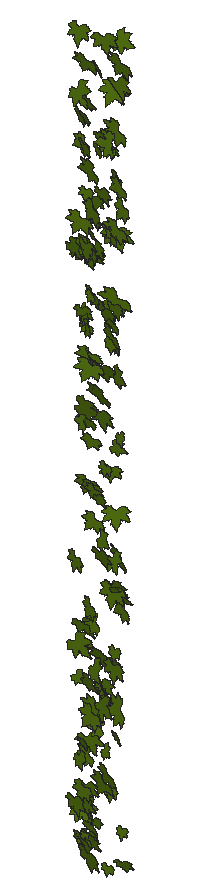
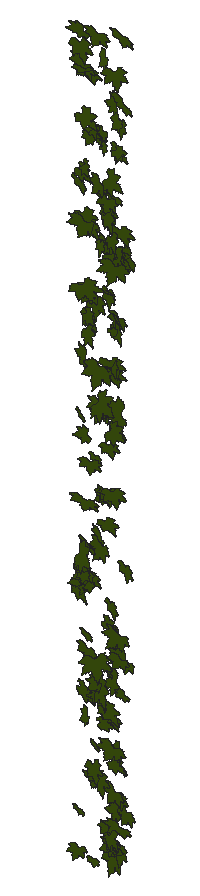
# SketchUp Ruby script. Lengths in inches.
U = 1.inch
M = Sketchup.active_model
def pt(a) = Geom::Point3d.new(a.map { |v| v * U })
def face(e, loops, mat)
  f = e.add_face(loops[0].map { |a| pt(a) })
  loops[1..].each { |l| e.add_face(l.map { |a| pt(a) }).erase! }
  f.material = f.back_material = mat if mat
  f
end
# faces: each face lists its corners as indices into pts; further lists are holes
def faces(e, pts, list, mat = nil) = list.each { |f| face(e, (f[0].is_a?(Array) ? f : [f]).map { |l| l.map { |i| pts[i] } }, mat) }
# xy, xz, yz: faces in a plane at the given z, y or x. An outline is a flat list of corners, or four numbers for a rectangle; further outlines are holes
def ring(l) = l.size == 4 ? [[l[0], l[1]], [l[2], l[1]], [l[2], l[3]], [l[0], l[3]]] : l.each_slice(2).to_a
def flat(e, list, mat, &to3) = list.each { |f| face(e, (f[0].is_a?(Array) ? f : [f]).map { |l| ring(l).map { |u, v| to3.(u, v) } }, mat) }
def xy(e, z, list, mat = nil) = flat(e, list, mat) { |x, y| [x, y, z] }
def xz(e, y, list, mat = nil) = flat(e, list, mat) { |x, z| [x, y, z] }
def yz(e, x, list, mat = nil) = flat(e, list, mat) { |y, z| [x, y, z] }
def lines(e, pts, list) = list.each { |a, b| e.add_line(pt(pts[a]), pt(pts[b])) }
# prism: a flat outline (further loops are holes) pulled along v
def prism(e, loops, v, mat = nil)
  f = face(e, loops, mat); d = Geom::Vector3d.new(v.map { |x| x * U })
  f.pushpull(f.normal.samedirection?(d) ? d.length : -d.length)
end
def box(e, o, s, mat = nil) = prism(e, [[o, [o[0] + s[0], o[1], o[2]], [o[0] + s[0], o[1] + s[1], o[2]], [o[0], o[1] + s[1], o[2]]]], [0, 0, s[2]], mat)
def at(x, y, z, deg = 0) = Geom::Transformation.translation(pt([x, y, z])) * Geom::Transformation.rotation(ORIGIN, Z_AXIS, deg.degrees)
def axes(o, x, y, z) = Geom::Transformation.new([*x, 0, *y, 0, *z, 0, *pt(o).to_a, 1])
def part(name) = M.definitions.add(name)
# library, detail: a bought-in or finely detailed component or shape, given as its bounding box
def library(name, o, s) = part(name).tap { |d| box(d.entities, o, s) }
def detail(e, o, s) = box(e.add_group.entities, o, s)
def put(e, d, t, mat = nil) = e.add_instance(d, t).tap { |i| i.material = mat if mat }
def group(e, t, mat = nil) = e.add_group.tap { |g| g.transformation = t; g.material = mat if mat }.entities
root = M.entities
M.materials.add("[Vegetation Blur 03]").color = [83, 114, 18]
c1 = part("ivy")
xy(c1.entities,0,[[0.782,0,0.786,0,0.787,0.005,0.789,0.009,0.821,0.072,0.875,0.147,1.001,0.272,1.073,0.331,1.137,0.363,1.178,0.379,1.223,0.384,1.272,0.383,1.311,0.374,1.36,0.355,1.399,0.334,1.491,0.285,1.541,0.244,1.583,0.199,1.617,0.15,1.64,0.128,1.662,0.115,1.717,0.105,1.745,0.093,1.784,0.054,1.819,0.057,1.854,0.064,1.882,0.075,1.896,0.074,1.91,0.071,1.937,0.063,1.964,0.053,1.99,0.038,2.016,0.015,2.034,0.002,2.04,0,2.038,0.003,2.036,0.007,2.033,0.038,2.036,0.068,2.045,0.1,2.055,0.116,2.064,0.123,2.077,0.129,2.088,0.129,2.106,0.132,2.118,0.13,2.179,0.132,2.207,0.133,2.225,0.133,2.242,0.138,2.22,0.162,2.207,0.186,2.206,0.213,2.212,0.236,2.228,0.262,2.247,0.274,2.298,0.283,2.355,0.294,2.37,0.296,2.376,0.295,2.377,0.3,2.377,0.303,2.385,0.329,2.411,0.37,2.426,0.392,2.449,0.407,2.511,0.426,2.561,0.444,2.619,0.466,2.589,0.469,2.561,0.476,2.501,0.5,2.449,0.516,2.424,0.523,2.401,0.535,2.377,0.556,2.372,0.568,2.36,0.575,2.268,0.586,2.225,0.592,2.207,0.599,2.194,0.61,2.143,0.65,2.13,0.664,2.122,0.682,2.123,0.7,2.13,0.719,2.148,0.75,2.17,0.781,2.195,0.807,2.221,0.828,2.284,0.874,2.291,0.88,2.288,0.887,2.276,0.9,2.267,0.916,2.265,0.933,2.273,0.967,2.292,1.002,2.313,1.03,2.334,1.054,2.348,1.067,2.358,1.074,2.363,1.076,2.362,1.081,2.35,1.094,2.347,1.11,2.35,1.143,2.359,1.18,2.385,1.254,2.415,1.324,2.448,1.393,2.45,1.4,2.446,1.398,2.44,1.394,2.427,1.383,2.402,1.36,2.376,1.339,2.345,1.324,2.305,1.309,2.282,1.303,2.273,1.306,2.245,1.294,2.212,1.287,2.187,1.291,2.163,1.301,2.142,1.316,2.134,1.327,2.124,1.325,2.09,1.292,2.053,1.259,2.014,1.234,1.973,1.215,1.954,1.21,1.931,1.208,1.909,1.212,1.893,1.22,1.879,1.233,1.872,1.248,1.867,1.281,1.864,1.319,1.821,1.258,1.773,1.197,1.726,1.141,1.698,1.121,1.679,1.116,1.666,1.117,1.647,1.122,1.632,1.129,1.62,1.141,1.617,1.154,1.617,1.219,1.621,1.254,1.623,1.268,1.623,1.281,1.618,1.314,1.606,1.346,1.603,1.375,1.607,1.403,1.603,1.467,1.599,1.499,1.605,1.525,1.614,1.552,1.629,1.577,1.635,1.589,1.629,1.587,1.618,1.582,1.596,1.566,1.581,1.556,1.568,1.552,1.557,1.55,1.545,1.553,1.531,1.562,1.522,1.572,1.504,1.591,1.486,1.611,1.474,1.631,1.457,1.666,1.455,1.684,1.457,1.698,1.452,1.715,1.444,1.728,1.424,1.754,1.419,1.772,1.423,1.786,1.434,1.819,1.444,1.848,1.446,1.855,1.44,1.861,1.43,1.867,1.386,1.904,1.349,1.948,1.326,1.973,1.31,1.995,1.288,2.048,1.284,2.153,1.287,2.254,1.284,2.255,1.282,2.253,1.278,2.247,1.274,2.237,1.266,2.216,1.226,2.125,1.208,2.076,1.184,2.033,1.155,1.984,1.135,1.942,1.111,1.899,1.083,1.861,1.053,1.85,1.059,1.83,1.061,1.809,1.056,1.79,1.049,1.767,1.04,1.749,1.018,1.733,0.994,1.726,0.942,1.734,0.95,1.6875,0.944,1.645,0.932,1.608,0.911,1.585,0.881,1.58,0.854,1.582,0.828,1.588,0.785,1.618,0.773,1.625,0.775,1.614,0.779,1.598,0.796,1.502,0.818,1.402,0.861,1.283,0.882,1.224,0.894,1.174,0.892,1.148,0.886,1.123,0.881,1.107,0.872,1.099,0.849,1.094,0.818,1.092,0.789,1.098,0.762,1.107,0.753,1.113,0.721,1.139,0.698,1.163,0.678,1.194,0.665,1.224,0.628,1.28,0.612,1.312,0.606,1.327,0.606,1.314,0.599,1.282,0.594,1.267,0.581,1.256,0.544,1.245,0.512,1.244,0.473,1.249,0.444,1.256,0.382,1.288,0.339,1.306,0.324,1.316,0.317,1.324,0.309,1.326,0.27,1.314,0.227,1.313,0.185,1.3125,0.152,1.317,0.122,1.328,0.092,1.345,0.073,1.353,0.079,1.338,0.092,1.308,0.117,1.249,0.13,1.215,0.139,1.164,0.147,1.148,0.157,1.136,0.163,1.122,0.174,1.086,0.177,1.067,0.182,1.054,0.186,1.043,0.191,1.038,0.211,1.028,0.237,1.005,0.25,0.974,0.253,0.96,0.25,0.944,0.242,0.914,0.243,0.906,0.249,0.902,0.26,0.894,0.289,0.88,0.307,0.873,0.322,0.862,0.364,0.799,0.403,0.738,0.431,0.709,0.439,0.691,0.441,0.678,0.4375,0.66,0.428,0.645,0.394,0.623,0.303,0.594,0.255,0.581,0.214,0.577,0.179,0.573,0.173,0.568,0.175,0.561,0.167,0.55,0.141,0.523,0.113,0.503,0.077,0.49,0.045,0.486,0.026,0.485,0.019,0.486,0.011,0.483,0,0.471,0.014,0.467,0.044,0.455,0.058,0.447,0.07,0.438,0.097,0.411,0.125,0.394,0.158,0.377,0.174,0.366,0.182,0.359,0.185,0.361,0.242,0.331,0.253,0.316,0.258,0.303,0.262,0.283,0.274,0.278,0.308,0.274,0.341,0.252,0.366,0.226,0.366,0.222,0.37,0.22,0.38,0.221,0.395,0.221,0.425,0.216,0.45,0.207,0.465,0.192,0.473,0.178,0.484,0.15,0.489,0.116,0.483,0.089,0.468,0.058,0.45,0.035,0.435,0.018,0.429,0.011,0.434,0.012,0.438,0.014,0.469,0.019,0.542,0.016,0.581,0.015,0.612,0.027,0.68,0.055,0.696,0.057,0.712,0.052,0.73,0.045,0.741,0.036,0.766,0.014]])
put(root,c1,axes([131.56,173.7,110.78],[0.17104,0.07406,0.23051],[0.28468,-0.03259,-0.13906],[0.00499,-0.6787,0.03183]),"[Vegetation Blur 03]")
put(root,c1,axes([131.55,173.7,117.41],[0.49502,-0.2424,-0.04719],[-0.06027,-0.00753,-0.41504],[-0.11656,-1.02555,0.0142]),"[Vegetation Blur 03]")
put(root,c1,axes([131.67,173.7,134.5625],[0.53942,-0.03341,-0.15907],[-0.19556,-0.07489,-0.43924],[-0.00287,-1.17788,0.03244]),"[Vegetation Blur 03]")
put(root,c1,axes([131.26,173.7,132.5],[0.30631,-0.15054,0.36025],[0.43855,-0.11732,-0.25607],[-0.08874,-1.09937,-0.022]),"[Vegetation Blur 03]")
put(root,c1,axes([132.41,173.7,124.4375],[0.12105,-0.13191,-0.28197],[-0.3442,0.10689,-0.10629],[-0.07075,-0.74572,0.03464]),"[Vegetation Blur 03]")
put(root,c1,axes([131.3125,173.7,104.97],[0.52242,-0.17809,0.13316],[0.16214,-0.04009,-0.43214],[-0.08844,-1.12553,-0.00568]),"[Vegetation Blur 03]")
put(root,c1,axes([132.25,173.7,138.55],[0.26106,-0.06742,-0.29363],[-0.35973,0.03582,-0.21432],[-0.03335,-0.91402,0.01326]),"[Vegetation Blur 03]")
put(root,c1,axes([131.875,173.7,139.82],[0.38591,-0.21569,-0.14541],[-0.15737,0.19687,-0.32414],[-0.13402,-0.85224,-0.03808]),"[Vegetation Blur 03]")
put(root,c1,axes([132.58,173.7,124.625],[0.1471,0.09742,-0.39347],[-0.48397,0.0748,-0.1176],[-0.02114,-1.03455,-0.04555]),"[Vegetation Blur 03]")
put(root,c1,axes([131.23,173.7,112.35],[0.3582,0.03063,0.42978],[0.52659,-0.05959,-0.29166],[-0.01559,-1.30923,0.02333]),"[Vegetation Blur 03]")
put(root,c1,axes([131.58,173.7,112.62],[0.36162,0.06548,0.17991],[0.22033,0.0215,-0.29621],[0.03262,-0.87124,0.00621]),"[Vegetation Blur 03]")
put(root,c1,axes([132.37,173.7,133.49],[0.37878,0.01189,-0.41383],[-0.50562,-0.09055,-0.30867],[0.03871,-1.29927,0.01773]),"[Vegetation Blur 03]")
put(root,c1,axes([131.89,173.7,142.52],[0.51764,0.02568,-0.18283],[-0.22378,0.14257,-0.41887],[-0.01616,-1.15189,-0.05592]),"[Vegetation Blur 03]")
put(root,c1,axes([131.82,173.7,103.34],[0.50401,-0.18357,-0.11952],[-0.1351,0.15116,-0.41597],[-0.10561,-1.06941,-0.03828]),"[Vegetation Blur 03]")
put(root,c1,axes([131.53,173.7,143.9375],[0.54024,-0.08088,0.09089],[0.10321,-0.19815,-0.43637],[-0.05739,-1.11765,0.07079]),"[Vegetation Blur 03]")
put(root,c1,axes([131.42,173.7,104.1],[0.37101,0.18964,0.31894],[0.39968,-0.06988,-0.30314],[0.03834,-1.10666,0.0738]),"[Vegetation Blur 03]")
put(root,c1,axes([132.75,173.7,137.29],[0.18125,0.04011,-0.45454],[-0.55361,0.15105,-0.14494],[-0.06386,-1.19573,-0.03356]),"[Vegetation Blur 03]")
put(root,c1,axes([132.35,173.7,129.625],[0.34504,-0.21965,-0.31495],[-0.37042,0.22285,-0.29474],[-0.152,-1.04167,0.00335]),"[Vegetation Blur 03]")
put(root,c1,axes([132.59,173.7,107.85],[0.21313,-0.07118,-0.35531],[-0.43534,0.04461,-0.17534],[-0.03471,-0.99647,0.01753]),"[Vegetation Blur 03]")
put(root,c1,axes([131.4,173.7,140.22],[0.34036,0.06769,0.40355],[0.48921,-0.24292,-0.26842],[-0.07909,-1.21115,0.07639]),"[Vegetation Blur 03]")
put(root,c1,axes([131.9,173.7,105.97],[0.51001,-0.14732,-0.08686],[-0.10909,-0.02593,-0.41973],[-0.06746,-1.07179,0.02209]),"[Vegetation Blur 03]")
put(root,c1,axes([132.4,173.7,134.11],[0.28115,-0.04858,-0.24392],[-0.28246,0.2397,-0.22437],[-0.10049,-0.80964,-0.05179]),"[Vegetation Blur 03]")
put(root,c1,axes([132,173.7,121.31],[0.48743,0.04761,-0.1367],[-0.16843,0.04371,-0.39762],[0.01495,-1.05971,-0.02254]),"[Vegetation Blur 03]")
put(root,c1,axes([132.43,173.7,127.74],[0.24639,-0.0769,-0.23479],[-0.27054,0.21951,-0.20041],[-0.10474,-0.7479,-0.03468]),"[Vegetation Blur 03]")
put(root,c1,axes([131.78,173.7,107.01],[0.30019,-0.07683,0.21744],[0.25164,-0.21034,-0.24309],[-0.09515,-0.7987,0.0431]),"[Vegetation Blur 03]")
put(root,c1,axes([132.72,173.7,104.45],[0.27997,-0.09905,-0.45822],[-0.54252,0.30141,-0.23104],[-0.15235,-1.25535,-0.01932]),"[Vegetation Blur 03]")
put(root,c1,axes([131.58,173.7,132.5],[0.59787,0.07047,0.08314],[0.09735,0.14687,-0.48587],[0.04553,-1.23935,-0.05285]),"[Vegetation Blur 03]")
put(root,c1,axes([132.0625,173.7,129.21],[0.05918,0.07636,0.27369],[0.32495,-0.20144,-0.03796],[-0.0908,-0.67116,0.04253]),"[Vegetation Blur 03]")
put(root,c1,axes([131.53,173.7,113.73],[0.50143,-0.04661,0.23263],[0.28578,0.12116,-0.40648],[0.00953,-1.18071,-0.05089]),"[Vegetation Blur 03]")
put(root,c1,axes([131.77,173.7,129.69],[0.45211,-0.0957,0.11404],[0.13937,-0.02195,-0.37092],[-0.04759,-0.97354,-0.00285]),"[Vegetation Blur 03]")
put(root,c1,axes([131.99,173.7,107.97],[0.28812,-0.17967,0.12477],[0.15963,0.01216,-0.24278],[-0.07425,-0.67108,-0.0378]),"[Vegetation Blur 03]")
put(root,c1,axes([132,173.7,138.25],[0.44121,-0.22953,-0.01023],[-0.00431,0.06987,-0.3705],[-0.11216,-0.9056,-0.026]),"[Vegetation Blur 03]")
put(root,c1,axes([131.86,173.7,102.72],[0.18512,0.00647,0.33943],[0.41367,-0.0999,-0.14998],[-0.04308,-0.93144,0.01844]),"[Vegetation Blur 03]")
put(root,c1,axes([132.13,173.7,135.79],[0.32765,-0.02489,0.01881],[0.02157,-0.07508,-0.26601],[-0.01455,-0.67173,0.02903]),"[Vegetation Blur 03]")
put(root,c1,axes([132.16,173.7,127.85],[0.50815,0.02983,-0.17456],[-0.21367,-0.02159,-0.41487],[0.01743,-1.13431,0.00331]),"[Vegetation Blur 03]")
put(root,c1,axes([132.49,173.7,129.24],[0.24945,-0.08617,-0.15972],[-0.19859,-0.02674,-0.20432],[-0.02483,-0.6519,0.02949]),"[Vegetation Blur 03]")
put(root,c1,axes([132.01,173.7,139.5625],[0.34754,-0.2147,0.09746],[0.13272,0.06991,-0.29103],[-0.08677,-0.75297,-0.05481]),"[Vegetation Blur 03]")
put(root,c1,axes([133.18,173.7,126.04],[0.15268,0.21133,-0.48982],[-0.60568,0.18355,-0.11329],[-0.06257,-1.26109,-0.09857]),"[Vegetation Blur 03]")
put(root,c1,axes([132.14,173.7,127.3],[0.55742,0.02012,-0.13001],[-0.15728,-0.13301,-0.4524],[0.0271,-1.18554,0.04855]),"[Vegetation Blur 03]")
put(root,c1,axes([131.89,173.7,133.24],[0.58629,-0.17522,0.04019],[0.04988,0.00183,-0.48347],[-0.08478,-1.21072,-0.00655]),"[Vegetation Blur 03]")
put(root,c1,axes([132.37,173.7,123.5],[0.38921,0.02788,-0.11804],[-0.14492,0.01541,-0.31769],[0.01009,-0.85429,-0.00958]),"[Vegetation Blur 03]")
put(root,c1,axes([132.71,173.7,135.32],[0.36249,-0.1648,-0.3565],[-0.41016,0.32061,-0.3011],[-0.17026,-1.12322,-0.03364]),"[Vegetation Blur 03]")
put(root,c1,axes([132.36,173.7,121.16],[0.40951,0.01971,-0.10583],[-0.13003,0.06915,-0.33309],[-0.00105,-0.88123,-0.0285]),"[Vegetation Blur 03]")
put(root,c1,axes([132.13,173.7,103.37],[0.37849,-0.06704,0.09137],[0.11442,0.06293,-0.30843],[-0.02244,-0.80977,-0.03153]),"[Vegetation Blur 03]")
put(root,c1,axes([131.76,173.7,108.03],[0.53376,0.03726,0.21952],[0.269,0.00727,-0.43585],[0.01776,-1.22992,0.00407]),"[Vegetation Blur 03]")
put(root,c1,axes([132.72,173.7,110.45],[0.42826,-0.11256,-0.35023],[-0.42906,0.04831,-0.35189],[-0.05529,-1.24664,0.01798]),"[Vegetation Blur 03]")
put(root,c1,axes([131.82,173.7,124.28],[0.20202,-0.16973,0.51163],[0.63222,0.07532,-0.16235],[0.00985,-1.35325,-0.07321]),"[Vegetation Blur 03]")
put(root,c1,axes([133.05,173.7,114.72],[0.19822,-0.13225,-0.36337],[-0.44645,0.06503,-0.16594],[-0.0552,-1.0008,0.03723]),"[Vegetation Blur 03]")
put(root,c1,axes([132.13,173.7,104.5],[0.13655,-0.05783,0.35944],[0.43753,-0.10617,-0.1134],[-0.05764,-0.9429,-0.00928]),"[Vegetation Blur 03]")
put(root,c1,axes([132.49,173.7,110.03],[0.51915,-0.17766,-0.225],[-0.28069,-0.03421,-0.42714],[-0.06834,-1.20911,0.04515]),"[Vegetation Blur 03]")
put(root,c1,axes([131.91,173.7,105.74],[0.52125,-0.12471,0.19571],[0.23821,-0.0569,-0.42827],[-0.06661,-1.17932,-0.00003]),"[Vegetation Blur 03]")
put(root,c1,axes([132.65,173.7,119.69],[0.40363,-0.02669,-0.22372],[-0.27442,-0.04788,-0.32887],[0.00236,-1.00289,0.02165]),"[Vegetation Blur 03]")
put(root,c1,axes([132.59,173.7,121.06],[0.38167,-0.01698,-0.15187],[-0.18516,0.0606,-0.31101],[-0.02031,-0.87168,-0.01866]),"[Vegetation Blur 03]")
put(root,c1,axes([132.47,173.7,115.37],[0.45232,-0.27078,-0.13351],[-0.16346,0.04761,-0.38403],[-0.13176,-0.98864,0.01808]),"[Vegetation Blur 03]")
put(root,c1,axes([132.62,173.7,130.86],[0.28246,-0.12607,-0.06429],[-0.08477,-0.04633,-0.23378],[-0.05266,-0.60166,0.03147]),"[Vegetation Blur 03]")
put(root,c1,axes([132.58,173.7,135.18],[0.47471,-0.2198,-0.23723],[-0.27334,0.21714,-0.39597],[-0.14555,-1.12467,-0.03009]),"[Vegetation Blur 03]")
put(root,c1,axes([133.07,173.7,127.25],[0.13027,0.06294,-0.24641],[-0.30303,0.06322,-0.10416],[-0.01626,-0.67369,-0.0328]),"[Vegetation Blur 03]")
put(root,c1,axes([132.01,173.7,102.72],[0.66178,-0.29714,0.00728],[0.02239,0.12543,-0.55031],[-0.14293,-1.35615,-0.0525]),"[Vegetation Blur 03]")
put(root,c1,axes([132.57,173.7,135.5],[0.50423,-0.25138,-0.23976],[-0.28758,0.12452,-0.42338],[-0.1361,-1.1944,0.00632]),"[Vegetation Blur 03]")
put(root,c1,axes([132.39,173.7,139.92],[0.06833,-0.14193,0.31087],[0.38368,-0.0807,-0.06197],[-0.05132,-0.79223,-0.04938]),"[Vegetation Blur 03]")
put(root,c1,axes([132.48,173.7,133.44],[0.499,-0.30069,-0.16614],[-0.19194,0.14146,-0.42426],[-0.16109,-1.09995,-0.00914]),"[Vegetation Blur 03]")
put(root,c1,axes([132.52,173.7,131.02],[0.4623,-0.23108,-0.11744],[-0.13279,0.12742,-0.38762],[-0.12523,-0.98816,-0.02252]),"[Vegetation Blur 03]")
put(root,c1,axes([132.3,173.7,135.6],[0.49002,-0.06773,0.03255],[0.04203,0.06603,-0.39982],[-0.03013,-1.00954,-0.02833]),"[Vegetation Blur 03]")
put(root,c1,axes([132.17,173.7,110.87],[0.2552,-0.21443,0.36363],[0.45118,-0.05704,-0.2162],[-0.07626,-1.05507,-0.06222]),"[Vegetation Blur 03]")
put(root,c1,axes([132.51,173.7,104.02],[0.2717,-0.01326,0.11926],[0.14597,0.06528,-0.22036],[0.00938,-0.63148,-0.02528]),"[Vegetation Blur 03]")
put(root,c1,axes([132.29,173.7,102.9],[0.29257,-0.13243,0.26003],[0.3239,0.04481,-0.23915],[-0.02726,-0.88901,-0.05079]),"[Vegetation Blur 03]")
put(root,c1,axes([133.08,173.7,111.5625],[0.44681,-0.13861,-0.40686],[-0.47518,0.33403,-0.36549],[-0.1651,-1.33648,-0.04915]),"[Vegetation Blur 03]")
put(root,c1,axes([133.5,173.7,109.41],[0.05855,-0.11186,-0.32035],[-0.39567,-0.06136,-0.0448],[0.02177,-0.81436,0.04738]),"[Vegetation Blur 03]")
put(root,c1,axes([132.75,173.7,112.84],[0.5883,0.12569,-0.22776],[-0.28567,0.25569,-0.4693],[0.00068,-1.31528,-0.113]),"[Vegetation Blur 03]")
put(root,c1,axes([132.97,173.7,138.33],[0.2858,-0.16556,-0.09391],[-0.1058,0.0991,-0.24194],[-0.0923,-0.62621,-0.01346]),"[Vegetation Blur 03]")
put(root,c1,axes([132.41,173.7,127.23],[0.67545,-0.01499,0.0047],[0.00705,0.26519,-0.54115],[-0.00605,-1.36446,-0.10523]),"[Vegetation Blur 03]")
put(root,c1,axes([133.05,173.7,133.39],[0.30779,-0.16022,-0.12096],[-0.12595,0.19898,-0.2549],[-0.11031,-0.67423,-0.04648]),"[Vegetation Blur 03]")
put(root,c1,axes([132.5625,173.7,111.51],[0.22572,0.02556,0.3673],[0.42622,-0.34586,-0.17068],[-0.14503,-0.97663,0.07006]),"[Vegetation Blur 03]")
put(root,c1,axes([132.84,173.7,138.75],[0.27595,-0.07999,0.10883],[0.13684,0.05207,-0.2251],[-0.02378,-0.62852,-0.0325]),"[Vegetation Blur 03]")
put(root,c1,axes([133,173.7,106.78],[0.5571,-0.15804,-0.2532],[-0.30286,0.14883,-0.45846],[-0.10211,-1.30372,-0.02164]),"[Vegetation Blur 03]")
put(root,c1,axes([132.73,173.7,132.92],[0.26922,-0.1042,0.25304],[0.30661,-0.09593,-0.2235],[-0.06845,-0.83952,-0.00587]),"[Vegetation Blur 03]")
put(root,c1,axes([132.85,173.7,142.38],[0.3403,-0.29163,0.09942],[0.13762,0.03874,-0.29588],[-0.12643,-0.74278,-0.05447]),"[Vegetation Blur 03]")
put(root,c1,axes([132.82,173.7,120.4],[0.28875,-0.1223,0.18363],[0.229,0.01809,-0.23796],[-0.04139,-0.75306,-0.03554]),"[Vegetation Blur 03]")
put(root,c1,axes([132.6,173.7,124.96],[0.63148,-0.16792,0.0994],[0.12538,0.04433,-0.51879],[-0.07597,-1.32267,-0.03001]),"[Vegetation Blur 03]")
put(root,c1,axes([132.86,173.7,110.93],[0.31712,0.01449,0.22059],[0.2693,0.0595,-0.25849],[0.0241,-0.85537,-0.01424]),"[Vegetation Blur 03]")
put(root,c1,axes([132.71,173.7,143.6875],[0.52799,0.03971,0.1403],[0.17249,-0.03446,-0.43082],[0.01316,-1.14211,0.01788]),"[Vegetation Blur 03]")
put(root,c1,axes([133,173.7,130.47],[0.55471,-0.15442,-0.09413],[-0.10485,0.16405,-0.45388],[-0.08911,-1.1543,-0.05191]),"[Vegetation Blur 03]")
put(root,c1,axes([132.72,173.7,117.86],[0.52924,-0.21641,0.13482],[0.17446,0.07604,-0.43695],[-0.08896,-1.13835,-0.05482]),"[Vegetation Blur 03]")
put(root,c1,axes([133.3125,173.7,107.23],[0.48731,-0.17978,-0.24983],[-0.29064,0.21865,-0.40235],[-0.12987,-1.16387,-0.037]),"[Vegetation Blur 03]")
put(root,c1,axes([133.03,173.7,118.02],[0.07963,0.08394,0.36792],[0.43963,-0.2386,-0.05481],[-0.10777,-0.91131,0.04824]),"[Vegetation Blur 03]")
put(root,c1,axes([133.71,173.7,134.43],[0.27575,-0.07071,-0.32237],[-0.38727,0.16418,-0.22631],[-0.08498,-0.9776,-0.01469]),"[Vegetation Blur 03]")
put(root,c1,axes([133.58,173.7,138.93],[0.3287,-0.1611,-0.24597],[-0.30329,0.03864,-0.27395],[-0.07054,-0.91688,0.03167]),"[Vegetation Blur 03]")
put(root,c1,axes([132.88,173.7,135.98],[0.42324,-0.15513,0.17492],[0.21736,0.00516,-0.3496],[-0.06611,-0.97622,-0.02964]),"[Vegetation Blur 03]")
put(root,c1,axes([134.03,173.7,139.27],[0.20332,-0.17652,-0.4378],[-0.54125,0.03497,-0.16965],[-0.04646,-1.17997,0.06046]),"[Vegetation Blur 03]")
put(root,c1,axes([133.26,173.7,110.13],[0.08923,-0.0651,0.22881],[0.28147,0.0622,-0.07033],[0.01942,-0.60224,-0.032]),"[Vegetation Blur 03]")
put(root,c1,axes([133.3,173.7,122.42],[0.35274,-0.11868,-0.02991],[-0.03922,-0.02703,-0.29129],[-0.05595,-0.72928,0.01566]),"[Vegetation Blur 03]")
put(root,c1,axes([133.29,173.7,107.58],[0.08406,0.07505,0.23958],[0.28752,-0.16835,-0.0589],[-0.06954,-0.60538,0.04608]),"[Vegetation Blur 03]")
put(root,c1,axes([134.29,173.7,118.12],[0.10735,0.13666,-0.49936],[-0.59338,0.3622,-0.06937],[-0.16335,-1.22594,-0.07616]),"[Vegetation Blur 03]")
put(root,c1,axes([133.4,173.7,102.17],[0.29298,-0.03076,-0.00517],[-0.00747,-0.046,-0.2387],[-0.01442,-0.60127,0.01853]),"[Vegetation Blur 03]")
put(root,c1,axes([133.86,173.7,129.08],[0.29122,-0.09132,-0.34949],[-0.40801,0.28097,-0.238],[-0.13739,-1.02797,-0.034]),"[Vegetation Blur 03]")
put(root,c1,axes([134,173.7,129.86],[0.15958,-0.02123,-0.31626],[-0.37905,0.17205,-0.12921],[-0.08118,-0.84504,-0.01836]),"[Vegetation Blur 03]")
put(root,c1,axes([132.88,173.7,109.62],[0.16056,0.04012,0.53459],[0.63688,-0.33645,-0.12344],[-0.15436,-1.34643,0.04677]),"[Vegetation Blur 03]")
put(root,c1,axes([133.23,173.7,122.21],[0.45127,0.0715,0.00789],[0.01018,-0.0128,-0.36935],[0.0346,-0.92876,0.0057]),"[Vegetation Blur 03]")
put(root,c1,axes([133.72,173.7,131.38],[0.53259,0.07407,-0.33493],[-0.4092,-0.06459,-0.43565],[0.04766,-1.38209,0.00241]),"[Vegetation Blur 03]")
put(root,c1,axes([134.09,173.7,139.9375],[0.36403,-0.06267,-0.40957],[-0.5016,0.04126,-0.29795],[-0.03412,-1.27511,0.01049]),"[Vegetation Blur 03]")
put(root,c1,axes([134.07,173.7,137.21],[0.19632,-0.0358,-0.23719],[-0.2774,0.19596,-0.15758],[-0.08838,-0.69459,-0.03223]),"[Vegetation Blur 03]")
put(root,c1,axes([133.58,173.7,138.38],[0.31483,-0.06922,0.03461],[0.04453,0.03834,-0.25772],[-0.03078,-0.65259,-0.01881]),"[Vegetation Blur 03]")
put(root,c1,axes([133.85,173.7,134.875],[0.46325,-0.03451,-0.29794],[-0.36488,0.02419,-0.37832],[-0.02045,-1.21347,0.00093]),"[Vegetation Blur 03]")
put(root,c1,axes([133.55,173.7,129.5],[0.58606,-0.32249,-0.17371],[-0.19607,0.18401,-0.49434],[-0.17725,-1.2698,-0.02752]),"[Vegetation Blur 03]")
put(root,c1,axes([133.62,173.7,106.16],[0.34421,-0.10508,0.04416],[0.04441,-0.1326,-0.28022],[-0.05969,-0.70465,0.04615]),"[Vegetation Blur 03]")
put(root,c1,axes([133.55,173.7,128.67],[0.3385,-0.12078,0.12895],[0.14584,-0.15588,-0.27795],[-0.08451,-0.75275,0.03687]),"[Vegetation Blur 03]")
put(root,c1,axes([133.34,173.7,116.47],[0.64834,-0.11558,0.00243],[-0.00125,-0.10055,-0.52962],[-0.05623,-1.33037,0.03982]),"[Vegetation Blur 03]")
put(root,c1,axes([134.33,173.7,137.03],[0.26205,-0.06963,-0.34462],[-0.42004,0.08964,-0.2156],[-0.05487,-1.01871,0.00458]),"[Vegetation Blur 03]")
put(root,c1,axes([133.55,173.7,141.82],[0.58164,-0.02914,-0.08506],[-0.10504,-0.22356,-0.46637],[0.00547,-1.19524,0.0893]),"[Vegetation Blur 03]")
put(root,c1,axes([134.47,173.7,111.02],[0.29249,-0.26424,-0.46367],[-0.56799,0.1604,-0.25303],[-0.12902,-1.30512,0.06278]),"[Vegetation Blur 03]")
put(root,c1,axes([133.86,173.7,116.43],[0.29824,-0.02143,-0.02343],[-0.02665,0.10046,-0.24043],[-0.01491,-0.60833,-0.03888]),"[Vegetation Blur 03]")
put(root,c1,axes([133.21,173.7,134.03],[0.60611,0.08882,0.16972],[0.20851,-0.00255,-0.49577],[0.04043,-1.31863,0.01239]),"[Vegetation Blur 03]")
put(root,c1,axes([133.375,173.7,120.07],[0.5345,0.11261,0.12686],[0.16236,-0.17388,-0.43135],[0.02823,-1.13219,0.07887]),"[Vegetation Blur 03]")
put(root,c1,axes([133.55,173.7,130.49],[0.44672,-0.11391,0.09884],[0.12385,0.0351,-0.3665],[-0.0489,-0.9518,-0.02535]),"[Vegetation Blur 03]")
put(root,c1,axes([133.8125,173.7,113.28],[0.33589,-0.10606,0.03492],[0.03467,-0.10992,-0.27466],[-0.05731,-0.68805,0.03849]),"[Vegetation Blur 03]")
put(root,c1,axes([133.5,173.7,112.54],[0.56428,-0.16916,0.04285],[0.04868,-0.06133,-0.46503],[-0.08453,-1.16458,0.01826]),"[Vegetation Blur 03]")
put(root,c1,axes([133.55,173.7,117.47],[0.29882,0.02623,0.28715],[0.33985,-0.26962,-0.23169],[-0.09199,-0.91085,0.07685]),"[Vegetation Blur 03]")
put(root,c1,axes([133.77,173.7,122.99],[0.12471,-0.00455,0.29508],[0.36083,0.05141,-0.10146],[0.0229,-0.78534,-0.00835]),"[Vegetation Blur 03]")
put(root,c1,axes([133.93,173.7,143.26],[0.56003,-0.11483,-0.22477],[-0.26984,0.13286,-0.4585],[-0.07841,-1.27735,-0.02748]),"[Vegetation Blur 03]")
put(root,c1,axes([133.5625,173.7,116.17],[0.35675,-0.1356,0.28151],[0.35114,0.1247,-0.28695],[-0.00453,-1.0135,-0.07297]),"[Vegetation Blur 03]")
put(root,c1,axes([134.49,173.7,115.94],[0.31943,-0.14813,-0.35105],[-0.42397,0.15166,-0.26703],[-0.10221,-1.09204,0.01053]),"[Vegetation Blur 03]")
put(root,c1,axes([133.8125,173.7,143.25],[0.0857,0.17777,0.39101],[0.48593,0.02942,-0.07304],[0.02949,-1.0011,0.06729]),"[Vegetation Blur 03]")
put(root,c1,axes([133.9,173.7,108.93],[0.26661,-0.22568,0.1584],[0.20153,-0.02212,-0.2309],[-0.09528,-0.67823,-0.04518]),"[Vegetation Blur 03]")
put(root,c1,axes([133.58,173.7,115.58],[0.27593,-0.17427,0.39331],[0.48854,0.16147,-0.21704],[0.02723,-1.13128,-0.09157]),"[Vegetation Blur 03]")
put(root,c1,axes([133.99,173.7,102.52],[0.36983,0.02306,0.04655],[0.05424,0.13467,-0.29755],[0.02088,-0.75816,-0.05144]),"[Vegetation Blur 03]")
put(root,c1,axes([133.51,173.7,141.69],[0.56787,-0.08069,0.24242],[0.2938,-0.10677,-0.464],[-0.05873,-1.31444,0.02281]),"[Vegetation Blur 03]")
put(root,c1,axes([134.03,173.7,126.59],[0.06006,-0.04189,0.40073],[0.47866,-0.22553,-0.0515],[-0.11129,-0.99263,-0.00521]),"[Vegetation Blur 03]")
put(root,c1,axes([134.15,173.7,123.97],[0.2323,-0.07315,0.16912],[0.19295,-0.17827,-0.18866],[-0.08352,-0.61528,0.03456]),"[Vegetation Blur 03]")
put(root,c1,axes([134.26,173.7,104.3],[0.28663,-0.07213,0.05383],[0.05877,-0.11436,-0.23255],[-0.04609,-0.59433,0.03821]),"[Vegetation Blur 03]")
put(root,c1,axes([134.32,173.7,136.08],[0.46163,-0.2581,-0.13642],[-0.17424,-0.01487,-0.3883],[-0.11538,-1.01019,0.04057]),"[Vegetation Blur 03]")
